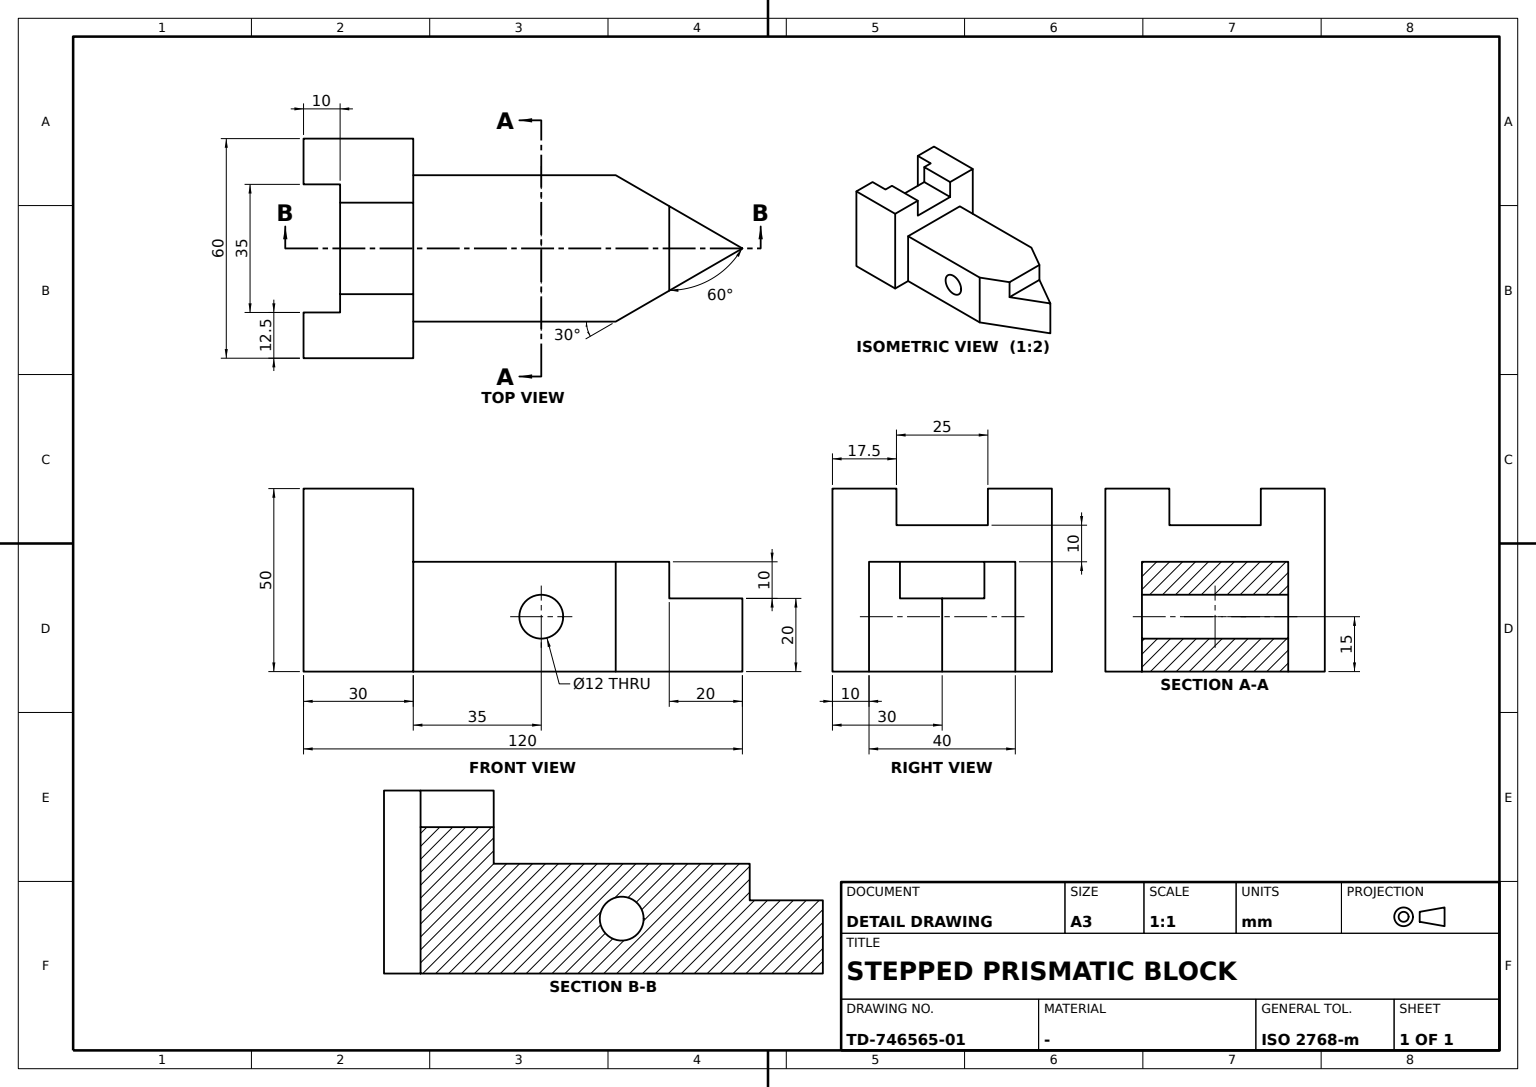
ISO-10303-21;
HEADER;
FILE_DESCRIPTION((''),'2;1');
FILE_NAME('','',(''),(''),'','','');
FILE_SCHEMA(('AUTOMOTIVE_DESIGN'));
ENDSEC;
DATA;
#1=APPLICATION_CONTEXT('');
#2=PRODUCT_CONTEXT('',#1,'mechanical');
#3=PRODUCT('','','',(#2));
#4=PRODUCT_DEFINITION_FORMATION('','',#3);
#5=PRODUCT_DEFINITION_CONTEXT('',#1,'design');
#6=PRODUCT_DEFINITION('','',#4,#5);
#7=PRODUCT_DEFINITION_SHAPE('','',#6);
#8=(LENGTH_UNIT()NAMED_UNIT(*)SI_UNIT(.MILLI.,.METRE.));
#9=(NAMED_UNIT(*)PLANE_ANGLE_UNIT()SI_UNIT($,.RADIAN.));
#10=(NAMED_UNIT(*)SI_UNIT($,.STERADIAN.)SOLID_ANGLE_UNIT());
#11=UNCERTAINTY_MEASURE_WITH_UNIT(LENGTH_MEASURE(1.E-05),#8,'distance_accuracy_value','');
#12=(GEOMETRIC_REPRESENTATION_CONTEXT(3)GLOBAL_UNCERTAINTY_ASSIGNED_CONTEXT((#11))GLOBAL_UNIT_ASSIGNED_CONTEXT((#8,#9,#10))REPRESENTATION_CONTEXT('',''));
#13=CARTESIAN_POINT('',(20.,85.358984,30.));
#14=VERTEX_POINT('',#13);
#15=CARTESIAN_POINT('',(20.,30.,30.));
#16=VERTEX_POINT('',#15);
#17=CARTESIAN_POINT('',(20.,57.679492,30.));
#18=DIRECTION('',(0.,-1.,0.));
#19=VECTOR('',#18,1000.);
#20=LINE('',#17,#19);
#21=EDGE_CURVE('',#14,#16,#20,.T.);
#22=ORIENTED_EDGE('',*,*,#21,.T.);
#23=CARTESIAN_POINT('',(20.,30.,0.));
#24=VERTEX_POINT('',#23);
#25=CARTESIAN_POINT('',(20.,30.,15.));
#26=DIRECTION('',(0.,0.,-1.));
#27=VECTOR('',#26,1000.);
#28=LINE('',#25,#27);
#29=EDGE_CURVE('',#16,#24,#28,.T.);
#30=ORIENTED_EDGE('',*,*,#29,.T.);
#31=CARTESIAN_POINT('',(20.,85.358984,0.));
#32=VERTEX_POINT('',#31);
#33=CARTESIAN_POINT('',(20.,57.679492,0.));
#34=LINE('',#33,#19);
#35=EDGE_CURVE('',#32,#24,#34,.T.);
#36=ORIENTED_EDGE('',*,*,#35,.F.);
#37=CARTESIAN_POINT('',(20.,85.358984,15.));
#38=DIRECTION('',(0.,0.,1.));
#39=VECTOR('',#38,1000.);
#40=LINE('',#37,#39);
#41=EDGE_CURVE('',#32,#14,#40,.T.);
#42=ORIENTED_EDGE('',*,*,#41,.T.);
#43=EDGE_LOOP('',(#22,#30,#36,#42));
#44=FACE_OUTER_BOUND('',#43,.T.);
#45=CARTESIAN_POINT('',(20.,71.,15.));
#46=VERTEX_POINT('',#45);
#47=CARTESIAN_POINT('',(20.,59.,15.));
#48=VERTEX_POINT('',#47);
#49=CARTESIAN_POINT('',(20.,65.,15.));
#50=DIRECTION('',(1.,0.,0.));
#51=DIRECTION('',(0.,1.,0.));
#52=AXIS2_PLACEMENT_3D('',#49,#50,#51);
#53=CIRCLE('',#52,6.);
#54=EDGE_CURVE('',#46,#48,#53,.T.);
#55=ORIENTED_EDGE('',*,*,#54,.F.);
#56=EDGE_CURVE('',#48,#46,#53,.T.);
#57=ORIENTED_EDGE('',*,*,#56,.F.);
#58=EDGE_LOOP('',(#55,#57));
#59=FACE_BOUND('',#58,.T.);
#60=CARTESIAN_POINT('',(20.,120.,30.));
#61=AXIS2_PLACEMENT_3D('',#60,#50,#18);
#62=PLANE('',#61);
#63=ADVANCED_FACE('',(#44,#59),#62,.T.);
#64=CARTESIAN_POINT('',(12.5,30.,40.));
#65=VERTEX_POINT('',#64);
#66=CARTESIAN_POINT('',(-12.5,30.,40.));
#67=VERTEX_POINT('',#66);
#68=CARTESIAN_POINT('',(0.,30.,40.));
#69=DIRECTION('',(-1.,0.,0.));
#70=VECTOR('',#69,1000.);
#71=LINE('',#68,#70);
#72=EDGE_CURVE('',#65,#67,#71,.T.);
#73=ORIENTED_EDGE('',*,*,#72,.F.);
#74=CARTESIAN_POINT('',(12.5,30.,50.));
#75=VERTEX_POINT('',#74);
#76=CARTESIAN_POINT('',(12.5,30.,45.));
#77=LINE('',#76,#27);
#78=EDGE_CURVE('',#75,#65,#77,.T.);
#79=ORIENTED_EDGE('',*,*,#78,.F.);
#80=CARTESIAN_POINT('',(30.,30.,50.));
#81=VERTEX_POINT('',#80);
#82=CARTESIAN_POINT('',(21.25,30.,50.));
#83=VECTOR('',#50,1000.);
#84=LINE('',#82,#83);
#85=EDGE_CURVE('',#75,#81,#84,.T.);
#86=ORIENTED_EDGE('',*,*,#85,.T.);
#87=CARTESIAN_POINT('',(30.,30.,0.));
#88=VERTEX_POINT('',#87);
#89=CARTESIAN_POINT('',(30.,30.,25.));
#90=LINE('',#89,#39);
#91=EDGE_CURVE('',#88,#81,#90,.T.);
#92=ORIENTED_EDGE('',*,*,#91,.F.);
#93=CARTESIAN_POINT('',(25.,30.,0.));
#94=LINE('',#93,#83);
#95=EDGE_CURVE('',#24,#88,#94,.T.);
#96=ORIENTED_EDGE('',*,*,#95,.F.);
#97=ORIENTED_EDGE('',*,*,#29,.F.);
#98=CARTESIAN_POINT('',(-20.,30.,30.));
#99=VERTEX_POINT('',#98);
#100=CARTESIAN_POINT('',(0.,30.,30.));
#101=LINE('',#100,#83);
#102=EDGE_CURVE('',#99,#16,#101,.T.);
#103=ORIENTED_EDGE('',*,*,#102,.F.);
#104=CARTESIAN_POINT('',(-20.,30.,0.));
#105=VERTEX_POINT('',#104);
#106=CARTESIAN_POINT('',(-20.,30.,15.));
#107=LINE('',#106,#27);
#108=EDGE_CURVE('',#99,#105,#107,.T.);
#109=ORIENTED_EDGE('',*,*,#108,.T.);
#110=CARTESIAN_POINT('',(-30.,30.,0.));
#111=VERTEX_POINT('',#110);
#112=CARTESIAN_POINT('',(-25.,30.,0.));
#113=LINE('',#112,#83);
#114=EDGE_CURVE('',#111,#105,#113,.T.);
#115=ORIENTED_EDGE('',*,*,#114,.F.);
#116=CARTESIAN_POINT('',(-30.,30.,50.));
#117=VERTEX_POINT('',#116);
#118=CARTESIAN_POINT('',(-30.,30.,25.));
#119=LINE('',#118,#39);
#120=EDGE_CURVE('',#111,#117,#119,.T.);
#121=ORIENTED_EDGE('',*,*,#120,.T.);
#122=CARTESIAN_POINT('',(-12.5,30.,50.));
#123=VERTEX_POINT('',#122);
#124=CARTESIAN_POINT('',(-21.25,30.,50.));
#125=LINE('',#124,#83);
#126=EDGE_CURVE('',#117,#123,#125,.T.);
#127=ORIENTED_EDGE('',*,*,#126,.T.);
#128=CARTESIAN_POINT('',(-12.5,30.,45.));
#129=LINE('',#128,#39);
#130=EDGE_CURVE('',#67,#123,#129,.T.);
#131=ORIENTED_EDGE('',*,*,#130,.F.);
#132=EDGE_LOOP('',(#73,#79,#86,#92,#96,#97,#103,#109,#115,#121,#127,#131));
#133=FACE_OUTER_BOUND('',#132,.T.);
#134=CARTESIAN_POINT('',(0.,30.,50.));
#135=AXIS2_PLACEMENT_3D('',#134,#18,#26);
#136=PLANE('',#135);
#137=ADVANCED_FACE('',(#133),#136,.F.);
#138=CARTESIAN_POINT('',(0.,120.,0.));
#139=VERTEX_POINT('',#138);
#140=CARTESIAN_POINT('',(10.,102.679492,0.));
#141=DIRECTION('',(0.5,-0.866025404,0.));
#142=VECTOR('',#141,1000.);
#143=LINE('',#140,#142);
#144=EDGE_CURVE('',#139,#32,#143,.T.);
#145=ORIENTED_EDGE('',*,*,#144,.F.);
#146=CARTESIAN_POINT('',(0.,120.,20.));
#147=VERTEX_POINT('',#146);
#148=CARTESIAN_POINT('',(0.,120.,10.));
#149=LINE('',#148,#27);
#150=EDGE_CURVE('',#147,#139,#149,.T.);
#151=ORIENTED_EDGE('',*,*,#150,.F.);
#152=CARTESIAN_POINT('',(11.547005,100.,20.));
#153=VERTEX_POINT('',#152);
#154=CARTESIAN_POINT('',(5.773503,110.,20.));
#155=LINE('',#154,#142);
#156=EDGE_CURVE('',#147,#153,#155,.T.);
#157=ORIENTED_EDGE('',*,*,#156,.T.);
#158=CARTESIAN_POINT('',(11.547005,100.,30.));
#159=VERTEX_POINT('',#158);
#160=CARTESIAN_POINT('',(11.547005,100.,25.));
#161=LINE('',#160,#27);
#162=EDGE_CURVE('',#159,#153,#161,.T.);
#163=ORIENTED_EDGE('',*,*,#162,.F.);
#164=CARTESIAN_POINT('',(15.773503,92.679492,30.));
#165=LINE('',#164,#142);
#166=EDGE_CURVE('',#159,#14,#165,.T.);
#167=ORIENTED_EDGE('',*,*,#166,.T.);
#168=ORIENTED_EDGE('',*,*,#41,.F.);
#169=EDGE_LOOP('',(#145,#151,#157,#163,#167,#168));
#170=FACE_OUTER_BOUND('',#169,.T.);
#171=CARTESIAN_POINT('',(0.,120.,30.));
#172=DIRECTION('',(0.866025404,0.5,0.));
#173=AXIS2_PLACEMENT_3D('',#171,#172,#141);
#174=PLANE('',#173);
#175=ADVANCED_FACE('',(#170),#174,.T.);
#176=CARTESIAN_POINT('',(-30.,0.,0.));
#177=VERTEX_POINT('',#176);
#178=CARTESIAN_POINT('',(-30.,15.,0.));
#179=VECTOR('',#51,1000.);
#180=LINE('',#178,#179);
#181=EDGE_CURVE('',#177,#111,#180,.T.);
#182=ORIENTED_EDGE('',*,*,#181,.F.);
#183=CARTESIAN_POINT('',(-30.,0.,50.));
#184=VERTEX_POINT('',#183);
#185=CARTESIAN_POINT('',(-30.,0.,25.));
#186=LINE('',#185,#27);
#187=EDGE_CURVE('',#184,#177,#186,.T.);
#188=ORIENTED_EDGE('',*,*,#187,.F.);
#189=CARTESIAN_POINT('',(-30.,15.,50.));
#190=LINE('',#189,#19);
#191=EDGE_CURVE('',#117,#184,#190,.T.);
#192=ORIENTED_EDGE('',*,*,#191,.F.);
#193=ORIENTED_EDGE('',*,*,#120,.F.);
#194=EDGE_LOOP('',(#182,#188,#192,#193));
#195=FACE_OUTER_BOUND('',#194,.T.);
#196=AXIS2_PLACEMENT_3D('',#176,#50,#51);
#197=PLANE('',#196);
#198=ADVANCED_FACE('',(#195),#197,.F.);
#199=CARTESIAN_POINT('',(-20.,71.,15.));
#200=VERTEX_POINT('',#199);
#201=CARTESIAN_POINT('',(-20.,59.,15.));
#202=VERTEX_POINT('',#201);
#203=CARTESIAN_POINT('',(-20.,65.,15.));
#204=AXIS2_PLACEMENT_3D('',#203,#69,#51);
#205=CIRCLE('',#204,6.);
#206=EDGE_CURVE('',#200,#202,#205,.T.);
#207=ORIENTED_EDGE('',*,*,#206,.F.);
#208=EDGE_CURVE('',#202,#200,#205,.T.);
#209=ORIENTED_EDGE('',*,*,#208,.F.);
#210=EDGE_LOOP('',(#207,#209));
#211=FACE_BOUND('',#210,.T.);
#212=ORIENTED_EDGE('',*,*,#108,.F.);
#213=CARTESIAN_POINT('',(-20.,85.358984,30.));
#214=VERTEX_POINT('',#213);
#215=CARTESIAN_POINT('',(-20.,57.679492,30.));
#216=LINE('',#215,#179);
#217=EDGE_CURVE('',#99,#214,#216,.T.);
#218=ORIENTED_EDGE('',*,*,#217,.T.);
#219=CARTESIAN_POINT('',(-20.,85.358984,0.));
#220=VERTEX_POINT('',#219);
#221=CARTESIAN_POINT('',(-20.,85.358984,15.));
#222=LINE('',#221,#27);
#223=EDGE_CURVE('',#214,#220,#222,.T.);
#224=ORIENTED_EDGE('',*,*,#223,.T.);
#225=CARTESIAN_POINT('',(-20.,57.679492,0.));
#226=LINE('',#225,#179);
#227=EDGE_CURVE('',#105,#220,#226,.T.);
#228=ORIENTED_EDGE('',*,*,#227,.F.);
#229=EDGE_LOOP('',(#212,#218,#224,#228));
#230=FACE_OUTER_BOUND('',#229,.T.);
#231=AXIS2_PLACEMENT_3D('',#98,#69,#51);
#232=PLANE('',#231);
#233=ADVANCED_FACE('',(#211,#230),#232,.T.);
#234=CARTESIAN_POINT('',(17.5,0.,0.));
#235=VERTEX_POINT('',#234);
#236=CARTESIAN_POINT('',(17.5,10.,0.));
#237=VERTEX_POINT('',#236);
#238=CARTESIAN_POINT('',(17.5,5.,0.));
#239=LINE('',#238,#179);
#240=EDGE_CURVE('',#235,#237,#239,.T.);
#241=ORIENTED_EDGE('',*,*,#240,.F.);
#242=CARTESIAN_POINT('',(17.5,0.,50.));
#243=VERTEX_POINT('',#242);
#244=CARTESIAN_POINT('',(17.5,0.,25.));
#245=LINE('',#244,#27);
#246=EDGE_CURVE('',#243,#235,#245,.T.);
#247=ORIENTED_EDGE('',*,*,#246,.F.);
#248=CARTESIAN_POINT('',(17.5,10.,50.));
#249=VERTEX_POINT('',#248);
#250=CARTESIAN_POINT('',(17.5,5.,50.));
#251=LINE('',#250,#179);
#252=EDGE_CURVE('',#243,#249,#251,.T.);
#253=ORIENTED_EDGE('',*,*,#252,.T.);
#254=CARTESIAN_POINT('',(17.5,10.,25.));
#255=LINE('',#254,#27);
#256=EDGE_CURVE('',#249,#237,#255,.T.);
#257=ORIENTED_EDGE('',*,*,#256,.T.);
#258=EDGE_LOOP('',(#241,#247,#253,#257));
#259=FACE_OUTER_BOUND('',#258,.T.);
#260=AXIS2_PLACEMENT_3D('',#248,#50,#18);
#261=PLANE('',#260);
#262=ADVANCED_FACE('',(#259),#261,.F.);
#263=CARTESIAN_POINT('',(-5.66,59.,15.));
#264=LINE('',#263,#70);
#265=EDGE_CURVE('',#48,#202,#264,.T.);
#266=ORIENTED_EDGE('',*,*,#265,.F.);
#267=ORIENTED_EDGE('',*,*,#56,.T.);
#268=CARTESIAN_POINT('',(-5.66,71.,15.));
#269=LINE('',#268,#70);
#270=EDGE_CURVE('',#46,#200,#269,.T.);
#271=ORIENTED_EDGE('',*,*,#270,.T.);
#272=ORIENTED_EDGE('',*,*,#206,.T.);
#273=EDGE_LOOP('',(#266,#267,#271,#272));
#274=FACE_OUTER_BOUND('',#273,.T.);
#275=CARTESIAN_POINT('',(-5.66,65.,15.));
#276=AXIS2_PLACEMENT_3D('',#275,#69,#51);
#277=CYLINDRICAL_SURFACE('',#276,6.);
#278=ADVANCED_FACE('',(#274),#277,.F.);
#279=ORIENTED_EDGE('',*,*,#162,.T.);
#280=CARTESIAN_POINT('',(-11.547005,100.,20.));
#281=VERTEX_POINT('',#280);
#282=CARTESIAN_POINT('',(0.,100.,20.));
#283=LINE('',#282,#70);
#284=EDGE_CURVE('',#153,#281,#283,.T.);
#285=ORIENTED_EDGE('',*,*,#284,.T.);
#286=CARTESIAN_POINT('',(-11.547005,100.,30.));
#287=VERTEX_POINT('',#286);
#288=CARTESIAN_POINT('',(-11.547005,100.,25.));
#289=LINE('',#288,#27);
#290=EDGE_CURVE('',#287,#281,#289,.T.);
#291=ORIENTED_EDGE('',*,*,#290,.F.);
#292=CARTESIAN_POINT('',(0.,100.,30.));
#293=LINE('',#292,#70);
#294=EDGE_CURVE('',#159,#287,#293,.T.);
#295=ORIENTED_EDGE('',*,*,#294,.F.);
#296=EDGE_LOOP('',(#279,#285,#291,#295));
#297=FACE_OUTER_BOUND('',#296,.T.);
#298=AXIS2_PLACEMENT_3D('',#292,#51,#26);
#299=PLANE('',#298);
#300=ADVANCED_FACE('',(#297),#299,.T.);
#301=ORIENTED_EDGE('',*,*,#223,.F.);
#302=CARTESIAN_POINT('',(-15.773503,92.679492,30.));
#303=DIRECTION('',(0.5,0.866025404,0.));
#304=VECTOR('',#303,1000.);
#305=LINE('',#302,#304);
#306=EDGE_CURVE('',#214,#287,#305,.T.);
#307=ORIENTED_EDGE('',*,*,#306,.T.);
#308=ORIENTED_EDGE('',*,*,#290,.T.);
#309=CARTESIAN_POINT('',(-5.773503,110.,20.));
#310=DIRECTION('',(-0.5,-0.866025404,0.));
#311=VECTOR('',#310,1000.);
#312=LINE('',#309,#311);
#313=EDGE_CURVE('',#147,#281,#312,.T.);
#314=ORIENTED_EDGE('',*,*,#313,.F.);
#315=ORIENTED_EDGE('',*,*,#150,.T.);
#316=CARTESIAN_POINT('',(-10.,102.679492,0.));
#317=LINE('',#316,#304);
#318=EDGE_CURVE('',#220,#139,#317,.T.);
#319=ORIENTED_EDGE('',*,*,#318,.F.);
#320=EDGE_LOOP('',(#301,#307,#308,#314,#315,#319));
#321=FACE_OUTER_BOUND('',#320,.T.);
#322=DIRECTION('',(0.866025404,-0.5,0.));
#323=AXIS2_PLACEMENT_3D('',#171,#322,#310);
#324=PLANE('',#323);
#325=ADVANCED_FACE('',(#321),#324,.F.);
#326=CARTESIAN_POINT('',(-17.5,10.,50.));
#327=VERTEX_POINT('',#326);
#328=CARTESIAN_POINT('',(-17.5,0.,50.));
#329=VERTEX_POINT('',#328);
#330=CARTESIAN_POINT('',(-17.5,5.,50.));
#331=LINE('',#330,#19);
#332=EDGE_CURVE('',#327,#329,#331,.T.);
#333=ORIENTED_EDGE('',*,*,#332,.F.);
#334=CARTESIAN_POINT('',(-12.5,10.,50.));
#335=VERTEX_POINT('',#334);
#336=CARTESIAN_POINT('',(-15.,10.,50.));
#337=LINE('',#336,#70);
#338=EDGE_CURVE('',#335,#327,#337,.T.);
#339=ORIENTED_EDGE('',*,*,#338,.F.);
#340=CARTESIAN_POINT('',(-12.5,20.,50.));
#341=LINE('',#340,#19);
#342=EDGE_CURVE('',#123,#335,#341,.T.);
#343=ORIENTED_EDGE('',*,*,#342,.F.);
#344=ORIENTED_EDGE('',*,*,#126,.F.);
#345=ORIENTED_EDGE('',*,*,#191,.T.);
#346=CARTESIAN_POINT('',(-23.75,0.,50.));
#347=LINE('',#346,#83);
#348=EDGE_CURVE('',#184,#329,#347,.T.);
#349=ORIENTED_EDGE('',*,*,#348,.T.);
#350=EDGE_LOOP('',(#333,#339,#343,#344,#345,#349));
#351=FACE_OUTER_BOUND('',#350,.T.);
#352=CARTESIAN_POINT('',(0.,0.,50.));
#353=AXIS2_PLACEMENT_3D('',#352,#26,#51);
#354=PLANE('',#353);
#355=ADVANCED_FACE('',(#351),#354,.F.);
#356=ORIENTED_EDGE('',*,*,#54,.T.);
#357=ORIENTED_EDGE('',*,*,#265,.T.);
#358=ORIENTED_EDGE('',*,*,#208,.T.);
#359=ORIENTED_EDGE('',*,*,#270,.F.);
#360=EDGE_LOOP('',(#356,#357,#358,#359));
#361=FACE_OUTER_BOUND('',#360,.T.);
#362=ADVANCED_FACE('',(#361),#277,.F.);
#363=CARTESIAN_POINT('',(-17.5,0.,0.));
#364=VERTEX_POINT('',#363);
#365=CARTESIAN_POINT('',(-17.5,0.,25.));
#366=LINE('',#365,#27);
#367=EDGE_CURVE('',#329,#364,#366,.T.);
#368=ORIENTED_EDGE('',*,*,#367,.T.);
#369=CARTESIAN_POINT('',(-17.5,10.,0.));
#370=VERTEX_POINT('',#369);
#371=CARTESIAN_POINT('',(-17.5,5.,0.));
#372=LINE('',#371,#179);
#373=EDGE_CURVE('',#364,#370,#372,.T.);
#374=ORIENTED_EDGE('',*,*,#373,.T.);
#375=CARTESIAN_POINT('',(-17.5,10.,25.));
#376=LINE('',#375,#27);
#377=EDGE_CURVE('',#327,#370,#376,.T.);
#378=ORIENTED_EDGE('',*,*,#377,.F.);
#379=ORIENTED_EDGE('',*,*,#332,.T.);
#380=EDGE_LOOP('',(#368,#374,#378,#379));
#381=FACE_OUTER_BOUND('',#380,.T.);
#382=AXIS2_PLACEMENT_3D('',#328,#69,#51);
#383=PLANE('',#382);
#384=ADVANCED_FACE('',(#381),#383,.F.);
#385=ORIENTED_EDGE('',*,*,#367,.F.);
#386=ORIENTED_EDGE('',*,*,#348,.F.);
#387=ORIENTED_EDGE('',*,*,#187,.T.);
#388=CARTESIAN_POINT('',(-23.75,0.,0.));
#389=LINE('',#388,#83);
#390=EDGE_CURVE('',#177,#364,#389,.T.);
#391=ORIENTED_EDGE('',*,*,#390,.T.);
#392=EDGE_LOOP('',(#385,#386,#387,#391));
#393=FACE_OUTER_BOUND('',#392,.T.);
#394=CARTESIAN_POINT('',(0.,0.,0.));
#395=AXIS2_PLACEMENT_3D('',#394,#51,#38);
#396=PLANE('',#395);
#397=ADVANCED_FACE('',(#393),#396,.F.);
#398=ORIENTED_EDGE('',*,*,#338,.T.);
#399=ORIENTED_EDGE('',*,*,#377,.T.);
#400=CARTESIAN_POINT('',(0.,10.,0.));
#401=LINE('',#400,#83);
#402=EDGE_CURVE('',#370,#237,#401,.T.);
#403=ORIENTED_EDGE('',*,*,#402,.T.);
#404=ORIENTED_EDGE('',*,*,#256,.F.);
#405=CARTESIAN_POINT('',(12.5,10.,50.));
#406=VERTEX_POINT('',#405);
#407=CARTESIAN_POINT('',(15.,10.,50.));
#408=LINE('',#407,#70);
#409=EDGE_CURVE('',#249,#406,#408,.T.);
#410=ORIENTED_EDGE('',*,*,#409,.T.);
#411=CARTESIAN_POINT('',(12.5,10.,40.));
#412=VERTEX_POINT('',#411);
#413=CARTESIAN_POINT('',(12.5,10.,45.));
#414=LINE('',#413,#27);
#415=EDGE_CURVE('',#406,#412,#414,.T.);
#416=ORIENTED_EDGE('',*,*,#415,.T.);
#417=CARTESIAN_POINT('',(-12.5,10.,40.));
#418=VERTEX_POINT('',#417);
#419=CARTESIAN_POINT('',(0.,10.,40.));
#420=LINE('',#419,#83);
#421=EDGE_CURVE('',#418,#412,#420,.T.);
#422=ORIENTED_EDGE('',*,*,#421,.F.);
#423=CARTESIAN_POINT('',(-12.5,10.,45.));
#424=LINE('',#423,#27);
#425=EDGE_CURVE('',#335,#418,#424,.T.);
#426=ORIENTED_EDGE('',*,*,#425,.F.);
#427=EDGE_LOOP('',(#398,#399,#403,#404,#410,#416,#422,#426));
#428=FACE_OUTER_BOUND('',#427,.T.);
#429=AXIS2_PLACEMENT_3D('',#326,#51,#50);
#430=PLANE('',#429);
#431=ADVANCED_FACE('',(#428),#430,.F.);
#432=CARTESIAN_POINT('',(30.,0.,50.));
#433=VERTEX_POINT('',#432);
#434=CARTESIAN_POINT('',(30.,0.,0.));
#435=VERTEX_POINT('',#434);
#436=CARTESIAN_POINT('',(30.,0.,25.));
#437=LINE('',#436,#27);
#438=EDGE_CURVE('',#433,#435,#437,.T.);
#439=ORIENTED_EDGE('',*,*,#438,.T.);
#440=CARTESIAN_POINT('',(30.,15.,0.));
#441=LINE('',#440,#179);
#442=EDGE_CURVE('',#435,#88,#441,.T.);
#443=ORIENTED_EDGE('',*,*,#442,.T.);
#444=ORIENTED_EDGE('',*,*,#91,.T.);
#445=CARTESIAN_POINT('',(30.,15.,50.));
#446=LINE('',#445,#19);
#447=EDGE_CURVE('',#81,#433,#446,.T.);
#448=ORIENTED_EDGE('',*,*,#447,.T.);
#449=EDGE_LOOP('',(#439,#443,#444,#448));
#450=FACE_OUTER_BOUND('',#449,.T.);
#451=AXIS2_PLACEMENT_3D('',#434,#50,#51);
#452=PLANE('',#451);
#453=ADVANCED_FACE('',(#450),#452,.T.);
#454=ORIENTED_EDGE('',*,*,#72,.T.);
#455=CARTESIAN_POINT('',(-12.5,20.,40.));
#456=LINE('',#455,#19);
#457=EDGE_CURVE('',#67,#418,#456,.T.);
#458=ORIENTED_EDGE('',*,*,#457,.T.);
#459=ORIENTED_EDGE('',*,*,#421,.T.);
#460=CARTESIAN_POINT('',(12.5,20.,40.));
#461=LINE('',#460,#19);
#462=EDGE_CURVE('',#65,#412,#461,.T.);
#463=ORIENTED_EDGE('',*,*,#462,.F.);
#464=EDGE_LOOP('',(#454,#458,#459,#463));
#465=FACE_OUTER_BOUND('',#464,.T.);
#466=AXIS2_PLACEMENT_3D('',#66,#26,#50);
#467=PLANE('',#466);
#468=ADVANCED_FACE('',(#465),#467,.F.);
#469=ORIENTED_EDGE('',*,*,#373,.F.);
#470=ORIENTED_EDGE('',*,*,#390,.F.);
#471=ORIENTED_EDGE('',*,*,#181,.T.);
#472=ORIENTED_EDGE('',*,*,#114,.T.);
#473=ORIENTED_EDGE('',*,*,#227,.T.);
#474=ORIENTED_EDGE('',*,*,#318,.T.);
#475=ORIENTED_EDGE('',*,*,#144,.T.);
#476=ORIENTED_EDGE('',*,*,#35,.T.);
#477=ORIENTED_EDGE('',*,*,#95,.T.);
#478=ORIENTED_EDGE('',*,*,#442,.F.);
#479=CARTESIAN_POINT('',(23.75,0.,0.));
#480=LINE('',#479,#83);
#481=EDGE_CURVE('',#235,#435,#480,.T.);
#482=ORIENTED_EDGE('',*,*,#481,.F.);
#483=ORIENTED_EDGE('',*,*,#240,.T.);
#484=ORIENTED_EDGE('',*,*,#402,.F.);
#485=EDGE_LOOP('',(#469,#470,#471,#472,#473,#474,#475,#476,#477,#478,#482,#483,#484));
#486=FACE_OUTER_BOUND('',#485,.T.);
#487=AXIS2_PLACEMENT_3D('',#394,#26,#51);
#488=PLANE('',#487);
#489=ADVANCED_FACE('',(#486),#488,.T.);
#490=ORIENTED_EDGE('',*,*,#415,.F.);
#491=CARTESIAN_POINT('',(12.5,20.,50.));
#492=LINE('',#491,#19);
#493=EDGE_CURVE('',#75,#406,#492,.T.);
#494=ORIENTED_EDGE('',*,*,#493,.F.);
#495=ORIENTED_EDGE('',*,*,#78,.T.);
#496=ORIENTED_EDGE('',*,*,#462,.T.);
#497=EDGE_LOOP('',(#490,#494,#495,#496));
#498=FACE_OUTER_BOUND('',#497,.T.);
#499=AXIS2_PLACEMENT_3D('',#64,#50,#38);
#500=PLANE('',#499);
#501=ADVANCED_FACE('',(#498),#500,.F.);
#502=ORIENTED_EDGE('',*,*,#284,.F.);
#503=ORIENTED_EDGE('',*,*,#156,.F.);
#504=ORIENTED_EDGE('',*,*,#313,.T.);
#505=EDGE_LOOP('',(#502,#503,#504));
#506=FACE_OUTER_BOUND('',#505,.T.);
#507=AXIS2_PLACEMENT_3D('',#146,#26,#18);
#508=PLANE('',#507);
#509=ADVANCED_FACE('',(#506),#508,.F.);
#510=ORIENTED_EDGE('',*,*,#493,.T.);
#511=ORIENTED_EDGE('',*,*,#409,.F.);
#512=ORIENTED_EDGE('',*,*,#252,.F.);
#513=CARTESIAN_POINT('',(23.75,0.,50.));
#514=LINE('',#513,#83);
#515=EDGE_CURVE('',#243,#433,#514,.T.);
#516=ORIENTED_EDGE('',*,*,#515,.T.);
#517=ORIENTED_EDGE('',*,*,#447,.F.);
#518=ORIENTED_EDGE('',*,*,#85,.F.);
#519=EDGE_LOOP('',(#510,#511,#512,#516,#517,#518));
#520=FACE_OUTER_BOUND('',#519,.T.);
#521=ADVANCED_FACE('',(#520),#354,.F.);
#522=ORIENTED_EDGE('',*,*,#438,.F.);
#523=ORIENTED_EDGE('',*,*,#515,.F.);
#524=ORIENTED_EDGE('',*,*,#246,.T.);
#525=ORIENTED_EDGE('',*,*,#481,.T.);
#526=EDGE_LOOP('',(#522,#523,#524,#525));
#527=FACE_OUTER_BOUND('',#526,.T.);
#528=ADVANCED_FACE('',(#527),#396,.F.);
#529=ORIENTED_EDGE('',*,*,#130,.T.);
#530=ORIENTED_EDGE('',*,*,#342,.T.);
#531=ORIENTED_EDGE('',*,*,#425,.T.);
#532=ORIENTED_EDGE('',*,*,#457,.F.);
#533=EDGE_LOOP('',(#529,#530,#531,#532));
#534=FACE_OUTER_BOUND('',#533,.T.);
#535=AXIS2_PLACEMENT_3D('',#122,#69,#26);
#536=PLANE('',#535);
#537=ADVANCED_FACE('',(#534),#536,.F.);
#538=ORIENTED_EDGE('',*,*,#294,.T.);
#539=ORIENTED_EDGE('',*,*,#306,.F.);
#540=ORIENTED_EDGE('',*,*,#217,.F.);
#541=ORIENTED_EDGE('',*,*,#102,.T.);
#542=ORIENTED_EDGE('',*,*,#21,.F.);
#543=ORIENTED_EDGE('',*,*,#166,.F.);
#544=EDGE_LOOP('',(#538,#539,#540,#541,#542,#543));
#545=FACE_OUTER_BOUND('',#544,.T.);
#546=AXIS2_PLACEMENT_3D('',#100,#26,#51);
#547=PLANE('',#546);
#548=ADVANCED_FACE('',(#545),#547,.F.);
#549=CLOSED_SHELL('',(#63,#137,#175,#198,#233,#262,#278,#300,#325,#355,#362,#384,#397,#431,#453,#468,#489,#501,#509,#521,#528,#537,#548));
#550=MANIFOLD_SOLID_BREP('',#549);
#551=ADVANCED_BREP_SHAPE_REPRESENTATION('',(#550),#12);
#552=SHAPE_DEFINITION_REPRESENTATION(#7,#551);
ENDSEC;
END-ISO-10303-21;
